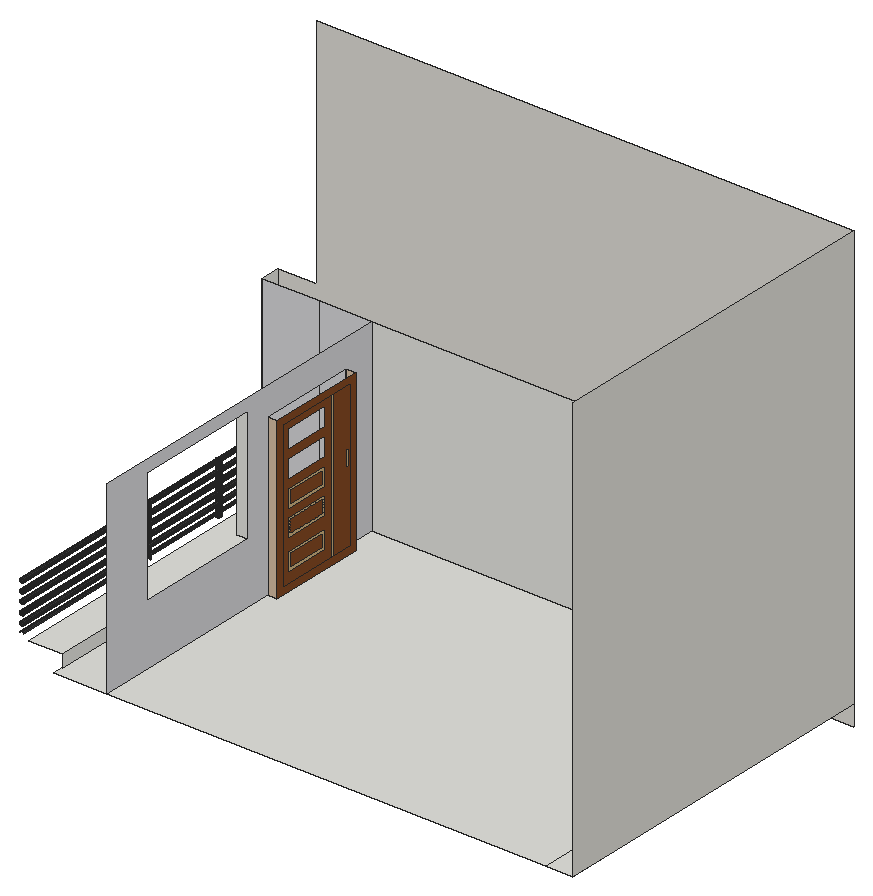
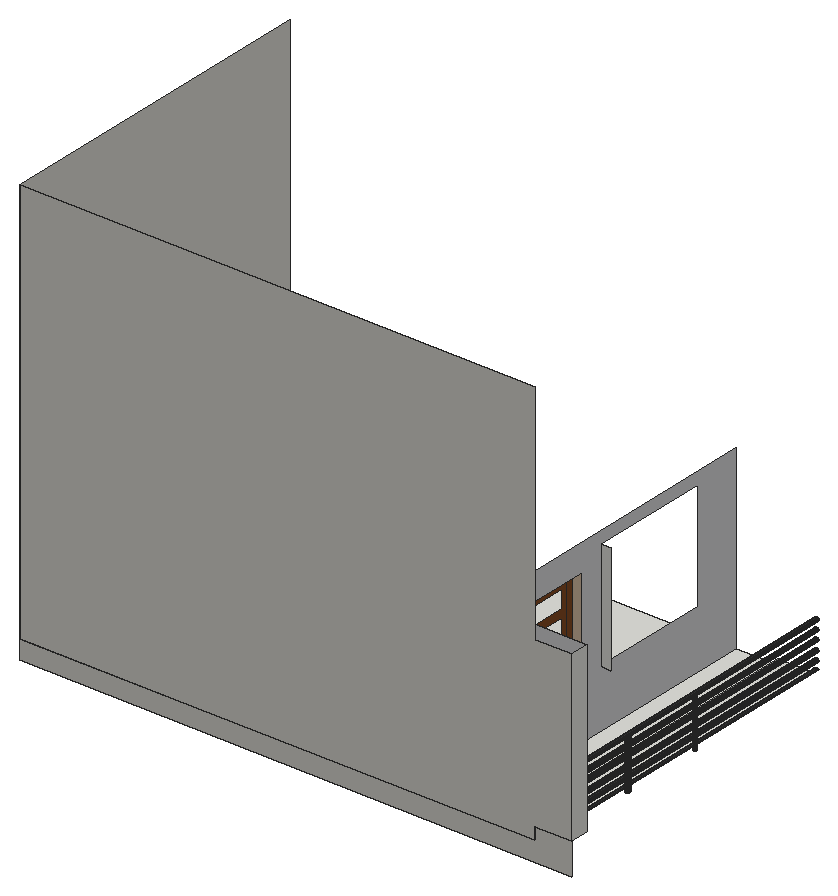
# SketchUp Ruby script. Lengths in inches.
U = 1.inch
M = Sketchup.active_model
def pt(a) = Geom::Point3d.new(a.map { |v| v * U })
def face(e, loops, mat)
  f = e.add_face(loops[0].map { |a| pt(a) })
  loops[1..].each { |l| e.add_face(l.map { |a| pt(a) }).erase! }
  f.material = f.back_material = mat if mat
  f
end
# faces: each face lists its corners as indices into pts; further lists are holes
def faces(e, pts, list, mat = nil) = list.each { |f| face(e, (f[0].is_a?(Array) ? f : [f]).map { |l| l.map { |i| pts[i] } }, mat) }
# xy, xz, yz: faces in a plane at the given z, y or x. An outline is a flat list of corners, or four numbers for a rectangle; further outlines are holes
def ring(l) = l.size == 4 ? [[l[0], l[1]], [l[2], l[1]], [l[2], l[3]], [l[0], l[3]]] : l.each_slice(2).to_a
def flat(e, list, mat, &to3) = list.each { |f| face(e, (f[0].is_a?(Array) ? f : [f]).map { |l| ring(l).map { |u, v| to3.(u, v) } }, mat) }
def xy(e, z, list, mat = nil) = flat(e, list, mat) { |x, y| [x, y, z] }
def xz(e, y, list, mat = nil) = flat(e, list, mat) { |x, z| [x, y, z] }
def yz(e, x, list, mat = nil) = flat(e, list, mat) { |y, z| [x, y, z] }
def lines(e, pts, list) = list.each { |a, b| e.add_line(pt(pts[a]), pt(pts[b])) }
# prism: a flat outline (further loops are holes) pulled along v
def prism(e, loops, v, mat = nil)
  f = face(e, loops, mat); d = Geom::Vector3d.new(v.map { |x| x * U })
  f.pushpull(f.normal.samedirection?(d) ? d.length : -d.length)
end
def box(e, o, s, mat = nil) = prism(e, [[o, [o[0] + s[0], o[1], o[2]], [o[0] + s[0], o[1] + s[1], o[2]], [o[0], o[1] + s[1], o[2]]]], [0, 0, s[2]], mat)
def at(x, y, z, deg = 0) = Geom::Transformation.translation(pt([x, y, z])) * Geom::Transformation.rotation(ORIGIN, Z_AXIS, deg.degrees)
def axes(o, x, y, z) = Geom::Transformation.new([*x, 0, *y, 0, *z, 0, *pt(o).to_a, 1])
def part(name) = M.definitions.add(name)
# library, detail: a bought-in or finely detailed component or shape, given as its bounding box
def library(name, o, s) = part(name).tap { |d| box(d.entities, o, s) }
def detail(e, o, s) = box(e.add_group.entities, o, s)
def put(e, d, t, mat = nil) = e.add_instance(d, t).tap { |i| i.material = mat if mat }
def group(e, t, mat = nil) = e.add_group.tap { |g| g.transformation = t; g.material = mat if mat }.entities
root = M.entities
M.materials.add("[Blinds Vertical Pattern]").color = [212, 212, 214]
M.materials.add("[Color M07]").color = [58, 58, 58]
M.materials.add("[Formica Laminate Light]").color = [213, 189, 164]
M.materials.add("[Terrazzo Tile Light]").color = [219, 217, 210]
M.materials.add("[Wood Cherry Original]").color = [130, 73, 35]
M.materials.add("[Wood Floor Light]").color = [204, 176, 127]
xy(root,18,[[509.21,483.625,509.21,779.875,53.375,779.875,53.375,797.6875,533.375,797.6875,533.375,483.625],[70.21,483.625,116.75,483.625,116.75,663.47,125.57,663.47,125.57,751.59,116.75,751.59,116.75,779.875,70.21,779.875],[116.75,483.625,116.75,663.47,125.57,663.47,125.57,751.59,116.75,751.59,116.75,779.875,509.21,779.875,509.21,483.625]])
xy(root,29.4375,[[40.07,492.63,70.21,779.875],[32.79,711.89,32.19,711.97,31.63,712.2,31.15,712.57,30.79,713.05,30.56,713.61,30.48,714.21,30.56,714.8,30.79,715.36,31.15,715.84,31.63,716.21,32.19,716.4375,32.79,716.52,33.39,716.4375,33.95,716.21,34.42,715.84,34.79,715.36,35.02,714.8,35.1,714.21,35.02,713.61,34.79,713.05,34.42,712.57,33.95,712.2,33.39,711.97],[18.625,779.875,53.375,797.6875]])
xy(root,75,[[32.79,711.89,33.39,711.97,33.95,712.2,34.42,712.57,34.79,713.05,35.02,713.61,35.1,714.21,35.02,714.8,34.79,715.36,34.42,715.84,33.95,716.21,33.39,716.4375,32.79,716.52,32.19,716.4375,31.63,716.21,31.15,715.84,30.79,715.36,30.56,714.8,30.48,714.21,30.56,713.61,30.79,713.05,31.15,712.57,31.63,712.2,32.19,711.97]],"[Color M07]")
xz(root,641.54,[[106.94,72.6,116.75,174.66]])
xz(root,663.47,[[116.75,18,125.57,160.59]],"[Formica Laminate Light]")
xz(root,751.59,[[116.75,18,125.57,160.59]],"[Formica Laminate Light]")
xz(root,779.875,[[53.375,18,70.21,29.4375],[116.75,18,509.21,185.6875]])
xz(root,779.875,[[70.21,18,116.75,185.6875],[[18.625,29.4375,70.21,185.6875],[34.16,39.43,33.69,39.49,33.25,39.67,32.88,39.96,32.59,40.34,32.41,40.77,32.35,41.24,32.41,41.71,32.59,42.15,32.88,42.52,33.25,42.8125,33.69,42.99,34.16,43.05,34.63,42.99,35.07,42.8125,35.44,42.52,35.73,42.15,35.91,41.71,35.97,41.24,35.91,40.77,35.73,40.34,35.44,39.96,35.07,39.67,34.63,39.49],[34.16,47.68,33.69,47.74,33.25,47.92,32.88,48.21,32.59,48.59,32.41,49.02,32.35,49.49,32.41,49.96,32.59,50.4,32.88,50.77,33.25,51.0625,33.69,51.24,34.16,51.3,34.63,51.24,35.07,51.0625,35.44,50.77,35.73,50.4,35.91,49.96,35.97,49.49,35.91,49.02,35.73,48.59,35.44,48.21,35.07,47.92,34.63,47.74],[34.16,56.74,33.69,56.8,33.25,56.99,32.88,57.27,32.59,57.65,32.41,58.09,32.35,58.55,32.41,59.02,32.59,59.46,32.88,59.84,33.25,60.125,33.69,60.31,34.16,60.37,34.63,60.31,35.07,60.125,35.44,59.84,35.73,59.46,35.91,59.02,35.97,58.55,35.91,58.09,35.73,57.65,35.44,57.27,35.07,56.99,34.63,56.8],[34.16,65.12,33.69,65.18,33.25,65.36,32.88,65.65,32.59,66.02,32.41,66.46,32.35,66.93,32.41,67.4,32.59,67.84,32.88,68.21,33.25,68.5,33.69,68.68,34.16,68.74,34.63,68.68,35.07,68.5,35.44,68.21,35.73,67.84,35.91,67.4,35.97,66.93,35.91,66.46,35.73,66.02,35.44,65.65,35.07,65.36,34.63,65.18],[34.16,73.8,33.69,73.87,33.25,74.05,32.88,74.34,32.59,74.71,32.41,75.15,32.35,75.62,32.41,76.09,32.59,76.52,32.88,76.9,33.25,77.1875,33.69,77.37,34.16,77.43,34.63,77.37,35.07,77.1875,35.44,76.9,35.73,76.52,35.91,76.09,35.97,75.62,35.91,75.15,35.73,74.71,35.44,74.34,35.07,74.05,34.63,73.87],[34.16,31.24,33.69,31.3,33.25,31.49,32.88,31.77,32.59,32.15,32.41,32.59,32.35,33.05,32.41,33.52,32.59,33.96,32.88,34.34,33.25,34.625,33.69,34.81,34.16,34.87,34.63,34.81,35.07,34.625,35.44,34.34,35.73,33.96,35.91,33.52,35.97,33.05,35.91,32.59,35.73,32.15,35.44,31.77,35.07,31.49,34.63,31.3]]],"[Blinds Vertical Pattern]")
xz(root,797.6875,[[18.625,0,18.625,29.4375,53.375,29.4375,53.375,18,533.375,18,533.375,0],[53.375,18,53.375,29.4375,18.625,29.4375,18.625,185.6875,53.375,185.6875,53.375,396.875,533.375,396.875,533.375,18]],"[Terrazzo Tile Light]")
yz(root,18.625,[[779.875,29.4375,797.6875,185.6875]])
yz(root,53.375,[[779.875,18,797.6875,29.4375]])
yz(root,70.21,[[492.63,18,779.875,29.4375]])
yz(root,116.75,[[[483.625,18,483.625,185.6875,779.875,185.6875,779.875,18,751.59,18,751.59,160.59,663.47,160.59,663.47,18],[528.53,72.6,641.54,174.66]]],"[Blinds Vertical Pattern]")
yz(root,125.57,[[[663.47,18,751.59,160.59],[669.49,24.02,745.57,154.57]],[[669.49,24.02,723.38,154.57],[675.02,132.1,716.58,148.91],[675.02,108.16,716.58,124.98],[675.02,84.35,716.58,101.16],[675.02,61.23,716.58,78.04],[675.02,34.1,716.58,50.91]],[[726.35,24.02,745.57,154.57],[740.27,89.05,743.39,103.8]],[677.42,36.5,714.18,48.51],[677.42,63.625,714.18,75.64],
  [677.42,86.75,714.18,98.76]],"[Wood Cherry Original]")
yz(root,125.57,[[723.38,24.02,726.35,154.57],[[675.02,34.1,716.58,50.91],[677.42,36.5,714.18,48.51]],[[675.02,61.23,716.58,78.04],[677.42,63.625,714.18,75.64]],[[675.02,84.35,716.58,101.16],[677.42,86.75,714.18,98.76]],[740.27,89.05,743.39,103.8]],"[Wood Floor Light]")
yz(root,533.375,[[483.625,18,797.6875,396.875]],"[Terrazzo Tile Light]")
p = [[31.63,636.65,29.4375],[31.15,636.28,29.4375],[31.15,636.28,76.375],[31.63,636.65,76.375],[34.42,636.28,29.4375],[33.95,636.65,29.4375],
  [33.95,636.65,76.375],[34.42,636.28,76.375],[32.19,636.875,29.4375],[32.19,636.875,76.375],[33.39,636.875,29.4375],[33.39,636.875,76.375],
  [32.79,636.96,29.4375],[32.79,636.96,76.375],[32.19,711.97,29.4375],[32.79,711.89,29.4375],[32.79,711.89,75],[32.19,711.97,75],
  [33.39,711.97,29.4375],[33.39,711.97,75],[31.63,712.2,29.4375],[31.63,712.2,75],[33.95,712.2,29.4375],[33.95,712.2,75],
  [31.15,712.57,29.4375],[31.15,712.57,75],[34.42,712.57,29.4375],[34.42,712.57,75],[30.79,713.05,29.4375],[30.79,713.05,75],
  [34.79,713.05,29.4375],[34.79,713.05,75],[30.56,713.61,29.4375],[30.56,713.61,75],[35.02,713.61,29.4375],[35.02,713.61,75],
  [30.48,714.21,29.4375],[30.48,714.21,75],[35.1,714.21,29.4375],[35.1,714.21,75],[30.56,714.8,29.4375],[30.56,714.8,75],
  [35.02,714.8,29.4375],[35.02,714.8,75],[30.79,715.36,29.4375],[30.79,715.36,75],[34.79,715.36,29.4375],[34.79,715.36,75],
  [31.15,715.84,29.4375],[31.15,715.84,75],[34.42,715.84,29.4375],[34.42,715.84,75],[31.63,716.21,29.4375],[31.63,716.21,75],
  [33.95,716.21,29.4375],[33.95,716.21,75],[32.19,716.4375,29.4375],[32.19,716.4375,75],[33.39,716.4375,29.4375],[33.39,716.4375,75],
  [32.79,716.52,29.4375],[32.79,716.52,75],[32.41,492.63,33.52],[32.59,492.63,33.96],[32.59,779.875,33.96],[32.41,779.875,33.52],
  [35.73,492.63,33.96],[35.91,492.63,33.52],[35.91,779.875,33.52],[35.73,779.875,33.96],[32.88,492.63,34.34],[32.88,779.875,34.34],
  [35.44,492.63,34.34],[35.44,779.875,34.34],[33.25,492.63,34.625],[33.25,779.875,34.625],[35.07,492.63,34.625],[35.07,779.875,34.625],
  [33.69,492.63,34.81],[33.69,779.875,34.81],[34.63,492.63,34.81],[34.63,779.875,34.81],[34.16,492.63,34.87],[34.16,779.875,34.87],
  [34.16,492.63,39.43],[33.69,492.63,39.49],[33.69,779.875,39.49],[34.16,779.875,39.43],[34.63,492.63,39.49],[34.63,779.875,39.49],
  [33.25,492.63,39.67],[33.25,779.875,39.67],[35.07,492.63,39.67],[35.07,779.875,39.67],[32.88,492.63,39.96],[32.88,779.875,39.96],
  [35.44,492.63,39.96],[35.44,779.875,39.96],[32.59,492.63,40.34],[32.59,779.875,40.34],[35.73,492.63,40.34],[35.73,779.875,40.34],
  [32.41,492.63,40.77],[32.41,779.875,40.77],[35.91,492.63,40.77],[35.91,779.875,40.77],[32.35,492.63,41.24],[32.35,779.875,41.24],
  [35.97,492.63,41.24],[35.97,779.875,41.24],[32.41,492.63,41.71],[32.41,779.875,41.71],[35.91,492.63,41.71],[35.91,779.875,41.71],
  [32.59,492.63,42.15],[32.59,779.875,42.15],[35.73,492.63,42.15],[35.73,779.875,42.15],[32.88,492.63,42.52],[32.88,779.875,42.52],
  [35.44,492.63,42.52],[35.44,779.875,42.52],[33.25,492.63,42.8125],[33.25,779.875,42.8125],[35.07,492.63,42.8125],[35.07,779.875,42.8125],
  [33.69,492.63,42.99],[33.69,779.875,42.99],[34.63,492.63,42.99],[34.63,779.875,42.99],[34.16,492.63,43.05],[34.16,779.875,43.05],
  [33.69,492.63,47.74],[33.25,492.63,47.92],[33.25,779.875,47.92],[33.69,779.875,47.74],[34.16,492.63,47.68],[34.16,779.875,47.68],
  [34.63,492.63,47.74],[34.63,779.875,47.74],[35.07,492.63,47.92],[35.07,779.875,47.92],[32.88,492.63,48.21],[32.88,779.875,48.21],
  [35.44,492.63,48.21],[35.44,779.875,48.21],[32.59,492.63,48.59],[32.59,779.875,48.59],[35.73,492.63,48.59],[35.73,779.875,48.59],
  [32.41,492.63,49.02],[32.41,779.875,49.02],[35.91,492.63,49.02],[35.91,779.875,49.02],[32.35,492.63,49.49],[32.35,779.875,49.49],
  [35.97,492.63,49.49],[35.97,779.875,49.49],[32.41,492.63,49.96],[32.41,779.875,49.96],[35.91,492.63,49.96],[35.91,779.875,49.96],
  [32.59,492.63,50.4],[32.59,779.875,50.4],[35.73,492.63,50.4],[35.73,779.875,50.4],[32.88,492.63,50.77],[32.88,779.875,50.77],
  [35.44,492.63,50.77],[35.44,779.875,50.77],[33.25,492.63,51.0625],[33.25,779.875,51.0625],[35.07,492.63,51.0625],[35.07,779.875,51.0625],
  [33.69,492.63,51.24],[33.69,779.875,51.24],[34.63,492.63,51.24],[34.63,779.875,51.24],[34.16,492.63,51.3],[34.16,779.875,51.3],
  [34.16,492.63,56.74],[33.69,492.63,56.8],[33.69,779.875,56.8],[34.16,779.875,56.74],[34.63,492.63,56.8],[34.63,779.875,56.8],
  [33.25,492.63,56.99],[33.25,779.875,56.99],[35.07,492.63,56.99],[35.07,779.875,56.99],[32.88,492.63,57.27],[32.88,779.875,57.27],
  [35.44,492.63,57.27],[35.44,779.875,57.27],[32.59,492.63,57.65],[32.59,779.875,57.65],[35.73,492.63,57.65],[35.73,779.875,57.65],
  [32.41,492.63,58.09],[32.41,779.875,58.09],[35.91,492.63,58.09],[35.91,779.875,58.09],[32.35,492.63,58.55],[32.35,779.875,58.55],
  [35.97,492.63,58.55],[35.97,779.875,58.55],[32.41,492.63,59.02],[32.41,779.875,59.02],[35.91,492.63,59.02],[35.91,779.875,59.02],
  [32.59,492.63,59.46],[32.59,779.875,59.46],[35.73,492.63,59.46],[35.73,779.875,59.46],[32.88,492.63,59.84],[32.88,779.875,59.84],
  [35.44,492.63,59.84],[35.44,779.875,59.84],[33.25,492.63,60.125],[33.25,779.875,60.125],[35.07,492.63,60.125],[35.07,779.875,60.125],
  [33.69,492.63,60.31],[33.69,779.875,60.31],[34.63,492.63,60.31],[34.63,779.875,60.31],[34.16,492.63,60.37],[34.16,779.875,60.37],
  [34.16,492.63,65.12],[33.69,492.63,65.18],[33.69,779.875,65.18],[34.16,779.875,65.12],[34.63,492.63,65.18],[34.63,779.875,65.18],
  [33.25,492.63,65.36],[33.25,779.875,65.36],[35.07,492.63,65.36],[35.07,779.875,65.36],[32.88,492.63,65.65],[32.88,779.875,65.65],
  [35.44,492.63,65.65],[35.44,779.875,65.65],[32.59,492.63,66.02],[32.59,779.875,66.02],[35.73,492.63,66.02],[35.73,779.875,66.02],
  [32.41,492.63,66.46],[32.41,779.875,66.46],[35.91,492.63,66.46],[35.91,779.875,66.46],[32.35,492.63,66.93],[32.35,779.875,66.93],
  [35.97,492.63,66.93],[35.97,779.875,66.93],[32.41,492.63,67.4],[32.41,779.875,67.4],[35.91,492.63,67.4],[35.91,779.875,67.4],
  [32.59,492.63,67.84],[32.59,779.875,67.84],[35.73,492.63,67.84],[35.73,779.875,67.84],[32.88,492.63,68.21],[32.88,779.875,68.21],
  [35.44,492.63,68.21],[35.44,779.875,68.21],[33.25,492.63,68.5],[33.25,779.875,68.5],[35.07,492.63,68.5],[35.07,779.875,68.5],
  [33.69,492.63,68.68],[33.69,779.875,68.68],[34.63,492.63,68.68],[34.63,779.875,68.68],[34.16,492.63,68.74],[34.16,779.875,68.74],
  [34.16,492.63,73.8],[33.69,492.63,73.87],[33.69,779.875,73.87],[34.16,779.875,73.8],[34.63,492.63,73.87],[34.63,779.875,73.87],
  [33.25,492.63,74.05],[33.25,779.875,74.05],[35.07,492.63,74.05],[35.07,779.875,74.05],[32.88,492.63,74.34],[32.88,779.875,74.34],
  [35.44,492.63,74.34],[35.44,779.875,74.34],[32.59,492.63,74.71],[32.59,779.875,74.71],[35.73,492.63,74.71],[35.73,779.875,74.71],
  [32.41,492.63,75.15],[32.41,779.875,75.15],[35.91,492.63,75.15],[35.91,779.875,75.15],[32.35,492.63,75.62],[32.35,779.875,75.62],
  [35.97,492.63,75.62],[35.97,779.875,75.62],[32.41,492.63,76.09],[32.41,779.875,76.09],[35.91,492.63,76.09],[35.91,779.875,76.09],
  [32.59,492.63,76.52],[32.59,779.875,76.52],[35.73,492.63,76.52],[35.73,779.875,76.52],[32.88,492.63,76.9],[32.88,779.875,76.9],
  [35.44,492.63,76.9],[35.44,779.875,76.9],[33.25,492.63,77.1875],[33.25,779.875,77.1875],[35.07,492.63,77.1875],[35.07,779.875,77.1875],
  [33.69,492.63,77.37],[33.69,779.875,77.37],[34.63,492.63,77.37],[34.63,779.875,77.37],[34.16,492.63,77.43],[34.16,779.875,77.43]]
faces(root,p,[[0,1,2,3],[4,5,6,7],[8,0,3,9],[5,10,11,6],[12,8,9,13],[10,12,13,11],[14,15,16,17],[15,18,19,16],
  [20,14,17,21],[18,22,23,19],[24,20,21,25],[22,26,27,23],[28,24,25,29],[26,30,31,27],[32,28,29,33],[30,34,35,31],
  [36,32,33,37],[34,38,39,35],[40,36,37,41],[38,42,43,39],[44,40,41,45],[42,46,47,43],[48,44,45,49],[46,50,51,47],
  [52,48,49,53],[50,54,55,51],[56,52,53,57],[54,58,59,55],[60,56,57,61],[58,60,61,59],[62,63,64,65],[66,67,68,69],
  [63,70,71,64],[72,66,69,73],[70,74,75,71],[76,72,73,77],[74,78,79,75],[80,76,77,81],[78,82,83,79],[82,80,81,83],
  [84,85,86,87],[88,84,87,89],[85,90,91,86],[92,88,89,93],[90,94,95,91],[96,92,93,97],[94,98,99,95],[100,96,97,101],
  [98,102,103,99],[104,100,101,105],[102,106,107,103],[108,104,105,109],[106,110,111,107],[112,108,109,113],[110,114,115,111],[116,112,113,117],
  [114,118,119,115],[120,116,117,121],[118,122,123,119],[124,120,121,125],[122,126,127,123],[128,124,125,129],[126,130,131,127],[130,128,129,131],
  [132,133,134,135],[136,132,135,137],[138,136,137,139],[140,138,139,141],[133,142,143,134],[144,140,141,145],[142,146,147,143],[148,144,145,149],
  [146,150,151,147],[152,148,149,153],[150,154,155,151],[156,152,153,157],[154,158,159,155],[160,156,157,161],[158,162,163,159],[164,160,161,165],
  [162,166,167,163],[168,164,165,169],[166,170,171,167],[172,168,169,173],[170,174,175,171],[176,172,173,177],[174,178,179,175],[178,176,177,179],
  [180,181,182,183],[184,180,183,185],[181,186,187,182],[188,184,185,189],[186,190,191,187],[192,188,189,193],[190,194,195,191],[196,192,193,197],
  [194,198,199,195],[200,196,197,201],[198,202,203,199],[204,200,201,205],[202,206,207,203],[208,204,205,209],[206,210,211,207],[212,208,209,213],
  [210,214,215,211],[216,212,213,217],[214,218,219,215],[220,216,217,221],[218,222,223,219],[224,220,221,225],[222,226,227,223],[226,224,225,227],
  [228,229,230,231],[232,228,231,233],[229,234,235,230],[236,232,233,237],[234,238,239,235],[240,236,237,241],[238,242,243,239],[244,240,241,245],
  [242,246,247,243],[248,244,245,249],[246,250,251,247],[252,248,249,253],[250,254,255,251],[256,252,253,257],[254,258,259,255],[260,256,257,261],
  [258,262,263,259],[264,260,261,265],[262,266,267,263],[268,264,265,269],[266,270,271,267],[272,268,269,273],[270,274,275,271],[274,272,273,275],
  [276,277,278,279],[280,276,279,281],[277,282,283,278],[284,280,281,285],[282,286,287,283],[288,284,285,289],[286,290,291,287],[292,288,289,293],
  [290,294,295,291],[296,292,293,297],[294,298,299,295],[300,296,297,301],[298,302,303,299],[304,300,301,305],[302,306,307,303],[308,304,305,309],
  [306,310,311,307],[312,308,309,313],[310,314,315,311],[316,312,313,317],[314,318,319,315],[320,316,317,321],[318,322,323,319],[322,320,321,323]],"[Color M07]")
